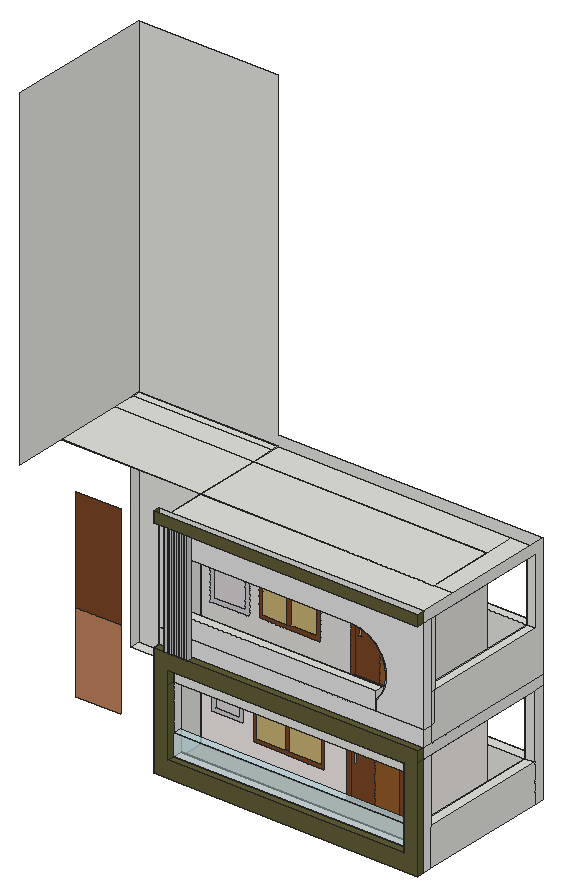
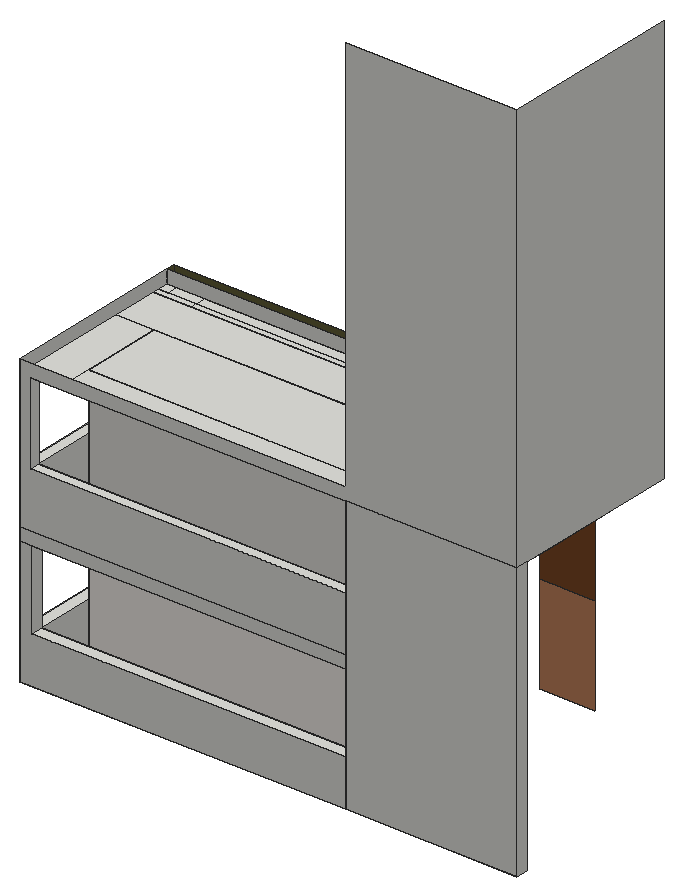
# SketchUp Ruby script. Lengths in inches.
U = 1.inch
M = Sketchup.active_model
def pt(a) = Geom::Point3d.new(a.map { |v| v * U })
def face(e, loops, mat)
  f = e.add_face(loops[0].map { |a| pt(a) })
  loops[1..].each { |l| e.add_face(l.map { |a| pt(a) }).erase! }
  f.material = f.back_material = mat if mat
  f
end
# faces: each face lists its corners as indices into pts; further lists are holes
def faces(e, pts, list, mat = nil) = list.each { |f| face(e, (f[0].is_a?(Array) ? f : [f]).map { |l| l.map { |i| pts[i] } }, mat) }
# xy, xz, yz: faces in a plane at the given z, y or x. An outline is a flat list of corners, or four numbers for a rectangle; further outlines are holes
def ring(l) = l.size == 4 ? [[l[0], l[1]], [l[2], l[1]], [l[2], l[3]], [l[0], l[3]]] : l.each_slice(2).to_a
def flat(e, list, mat, &to3) = list.each { |f| face(e, (f[0].is_a?(Array) ? f : [f]).map { |l| ring(l).map { |u, v| to3.(u, v) } }, mat) }
def xy(e, z, list, mat = nil) = flat(e, list, mat) { |x, y| [x, y, z] }
def xz(e, y, list, mat = nil) = flat(e, list, mat) { |x, z| [x, y, z] }
def yz(e, x, list, mat = nil) = flat(e, list, mat) { |y, z| [x, y, z] }
def lines(e, pts, list) = list.each { |a, b| e.add_line(pt(pts[a]), pt(pts[b])) }
# prism: a flat outline (further loops are holes) pulled along v
def prism(e, loops, v, mat = nil)
  f = face(e, loops, mat); d = Geom::Vector3d.new(v.map { |x| x * U })
  f.pushpull(f.normal.samedirection?(d) ? d.length : -d.length)
end
def box(e, o, s, mat = nil) = prism(e, [[o, [o[0] + s[0], o[1], o[2]], [o[0] + s[0], o[1] + s[1], o[2]], [o[0], o[1] + s[1], o[2]]]], [0, 0, s[2]], mat)
def at(x, y, z, deg = 0) = Geom::Transformation.translation(pt([x, y, z])) * Geom::Transformation.rotation(ORIGIN, Z_AXIS, deg.degrees)
def axes(o, x, y, z) = Geom::Transformation.new([*x, 0, *y, 0, *z, 0, *pt(o).to_a, 1])
def part(name) = M.definitions.add(name)
# library, detail: a bought-in or finely detailed component or shape, given as its bounding box
def library(name, o, s) = part(name).tap { |d| box(d.entities, o, s) }
def detail(e, o, s) = box(e.add_group.entities, o, s)
def put(e, d, t, mat = nil) = e.add_instance(d, t).tap { |i| i.material = mat if mat }
def group(e, t, mat = nil) = e.add_group.tap { |g| g.transformation = t; g.material = mat if mat }.entities
root = M.entities
M.materials.add("[0057_DarkKhaki]").color = [96, 93, 54]
M.materials.add("[Blinds Cellular White]").color = [217, 211, 213]
M.materials.add("[Carpet Diamond Yellow]").color = [226, 217, 124]
M.materials.add("[Carpet Pattern Leaf Squares Tan]").color = [181, 154, 125]
M.materials.add("[Polished Concrete New]").color = [200, 200, 203]
M.materials.add("[Polished Concrete Old]").color = [229, 229, 229]
M.materials.add("[Terrazzo Tile Accent]").color = [224, 221, 217]
M.materials.add("[Translucent Glass Safety]").color = [204, 235, 244]
M.materials["[Translucent Glass Safety]"].alpha = 0.5
M.materials.add("[White Square Tile]").color = [240, 234, 230]
M.materials.add("[Window Covering 02]").color = [199, 178, 115]
M.materials.add("[Wood Floor Light]").color = [204, 176, 127]
M.materials.add("[Wood Floor Parquet]").color = [145, 89, 39]
M.materials.add("[Wood Veneer 01]").color = [120, 70, 37]
M.materials.add("[Wood Veneer 02]").color = [190, 128, 91]
xy(root,354.875,[[386.67,294.37,424.8,314.12],[424.8,294.37,1062.63,314.12],[1062.63,294.37,1099.23,314.12],[386.67,314.12,424.8,338.96],[424.8,314.12,1062.63,338.96],
  [1062.63,314.12,1099.23,338.96],[1072.84,338.96,1072.84,688.57,386.67,688.57,386.67,714.96,1099.23,714.96,1099.23,338.96],[386.67,454.33,997.73,653.02],[11.875,688.57,386.67,714.96]])
xy(root,354.875,[[386.67,338.96,1072.84,338.96,1072.84,688.57,386.67,688.57,386.67,653.02,997.73,653.02,997.73,454.33,386.67,454.33]],"[Carpet Pattern Leaf Squares Tan]")
xy(root,398.5625,[[424.8,314.12,1062.63,338.96]])
xy(root,398.5625,[[424.8,294.37,1062.63,314.12]],"[0057_DarkKhaki]")
xy(root,454.8125,[[424.8,314.12,1062.63,338.96]],"[Translucent Glass Safety]")
xy(root,457.5,[[1072.84,338.96,1099.23,688.57],[386.67,688.57,1072.84,714.96]])
xy(root,579.75,[[424.8,314.12,1062.63,338.96]])
xy(root,616.5625,[[424.8,314.12,1062.63,338.96]])
xy(root,616.5625,[[424.8,294.37,1062.63,314.12]],"[0057_DarkKhaki]")
xy(root,629.6875,[[386.67,338.96,386.67,454.33,997.73,454.33,997.73,714.96,1072.84,714.96,1072.84,688.57,1099.23,688.57,1099.23,338.96],[386.67,454.33,997.73,653.02],[386.67,653.02,997.73,714.96]])
xy(root,657,[[415.15,294.37,424.7,307.59],[427.33,294.37,436.89,307.59],[440.83,294.37,450.39,307.59],[454.9,294.37,464.45,307.59],[467.49,294.37,477.04,307.59],
  [386.67,314.12,386.67,338.96,1075.67,337.88,1099.23,337.88,1099.23,314.12],[1075.67,337.88,1075.67,693,386.67,693,386.67,714.96,1099.23,714.96,1099.23,337.88],[386.67,452.96,1015.29,631.96]])
xy(root,657,[[386.67,294.37,415.15,294.37,415.15,307.59,424.7,307.59,424.7,294.37,427.33,294.37,427.33,307.59,436.89,307.59,436.89,294.37,440.83,294.37,440.83,307.59,450.39,307.59,450.39,294.37,454.9,294.37,454.9,307.59,464.45,307.59,464.45,294.37,467.49,294.37,467.49,307.59,477.04,307.59,477.04,294.37,1099.23,294.37,1099.23,314.12,386.67,314.12]],"[0057_DarkKhaki]")
xy(root,657,[[1075.67,337.88,1075.67,693,386.67,693,386.67,631.96,1015.29,631.96,1015.29,452.96,386.67,452.96,386.67,338.96]],"[Carpet Diamond Yellow]")
xy(root,699.68,[[386.67,314.12,427.13,337.88],[427.13,314.12,903.88,337.98],[903.88,314.12,970.81,337.88],[970.81,314.12,1099.23,337.88],[386.67,337.88,386.67,338.96,427.13,338.89,427.13,337.88],
  [1075.67,337.88,903.88,338.15,903.88,351.68,1099.23,351.68,1099.23,337.88],[903.88,337.88,903.88,338.15,1075.67,337.88],[427.13,338.89,386.67,338.96,386.67,351.68,427.13,351.68]])
xy(root,748.74,[[410.19,314.12,970.81,314.12,970.81,337.88,903.88,337.88,903.88,337.98,427.13,337.98,427.13,337.88,410.19,337.88]])
xy(root,779.4375,[[1075.67,337.88,1099.23,693],[386.67,693,1075.67,714.96]])
xy(root,889.43,[[410.19,314.12,903.88,337.88],[427.13,337.88,903.88,337.98],[427.13,337.98,903.88,351.68]])
xy(root,958.5625,[[386.67,294.37,386.67,314.12,1015.29,314.12,1015.29,294.37,477.04,294.37,477.04,307.59,467.49,307.59,467.49,294.37,464.45,294.37,464.45,307.59,454.9,307.59,454.9,294.37,450.39,294.37,450.39,307.59,440.83,307.59,440.83,294.37,436.89,294.37,436.89,307.59,427.33,307.59,427.33,294.37,424.7,294.37,424.7,307.59,415.15,307.59,415.15,294.37],[415.15,294.37,424.7,307.59],[427.33,294.37,436.89,307.59],[440.83,294.37,450.39,307.59],[454.9,294.37,464.45,307.59],
  [467.49,294.37,477.04,307.59],[1015.29,294.37,1075.67,314.12],[1075.67,294.37,1099.23,314.12],[386.67,314.12,1015.29,314.12,1015.29,337.98,386.67,338.96],[1015.29,314.12,1015.29,337.98,1075.67,337.88,1075.67,314.12],
  [1075.67,314.12,1099.23,337.88],[1075.67,337.88,1099.23,337.88,1099.23,351.68,1015.29,351.68,1015.29,337.98],[1015.29,337.98,386.67,338.96,386.67,351.68,1015.29,351.68],[386.67,351.68,1099.23,452.96],[11.875,452.96,386.67,454.33],
  [386.67,452.96,1015.29,631.96],[1015.29,452.96,1015.29,714.96,1075.67,714.96,1075.67,693,1099.23,693,1099.23,452.96],[11.875,454.33,386.67,631.96],[11.875,631.96,386.67,693],[386.67,631.96,1015.29,714.96],
  [11.875,693,386.67,714.96]])
xz(root,294.37,[[[386.67,354.875,1099.23,657],[424.8,398.5625,1062.63,616.5625]],[386.67,958.5625,1099.23,986.8125]],"[0057_DarkKhaki]")
xz(root,294.37,[[415.15,657,424.7,958.5625],[427.33,657,436.89,958.5625],[440.83,657,450.39,958.5625],[454.9,657,464.45,958.5625],[467.49,657,477.04,958.5625]],"[Polished Concrete New]")
xz(root,307.59,[[415.15,657,424.7,958.5625],[427.33,657,436.89,958.5625],[440.83,657,450.39,958.5625],[454.9,657,464.45,958.5625],[467.49,657,477.04,958.5625]])
xz(root,314.12,[[424.8,579.75,1062.63,616.5625],[386.67,958.5625,1099.23,986.8125]])
xz(root,314.12,[[386.67,657,1099.23,699.68],[386.67,699.68,970.81,699.68,970.81,748.74,410.19,748.74,410.19,889.43,903.88,889.43,928.43,886.2,951.31,876.72,970.96,861.64,986.04,841.99,995.52,819.11,998.75,794.55,995.52,770,986.04,747.12,970.96,727.47,970.81,727.35,970.81,699.68,1099.23,699.68,1099.23,958.5625,386.67,958.5625]],"[Polished Concrete Old]")
xz(root,314.12,[[424.8,398.5625,1062.63,454.8125]],"[Translucent Glass Safety]")
xz(root,314.12,[[163.125,665.78,282.875,947.1]],"[Wood Veneer 01]")
xz(root,314.12,[[163.125,450.91,282.875,665.78]],"[Wood Veneer 02]")
xz(root,337.88,[[1075.67,657,1099.23,699.68],[903.88,699.68,903.88,748.74,970.81,748.74,970.81,727.35,951.31,712.39,928.44,702.91,928.43,702.91],[903.88,699.68,928.43,702.91,970.81,702.91,970.81,699.68],[1075.67,699.68,1099.23,779.4375],[928.44,702.91,951.31,712.39,970.81,727.35,970.81,702.91],
  [410.19,748.74,427.13,889.43],[1075.67,779.4375,1099.23,958.5625]])
xz(root,337.98,[[427.13,699.68,903.88,748.74]])
xz(root,338.96,[[386.67,354.875,424.8,629.6875],[424.8,354.875,1062.63,398.5625],[1062.63,354.875,1072.84,629.6875],[1072.84,354.875,1099.23,457.5],[1072.84,457.5,1099.23,629.6875],
  [424.8,579.75,1062.63,616.5625],[424.8,616.5625,1062.63,629.6875]])
xz(root,338.96,[[424.8,398.5625,1062.63,454.8125]],"[Translucent Glass Safety]")
xz(root,351.68,[[386.67,699.68,386.67,958.5625,1099.23,958.5625,1099.23,699.68,903.88,699.68,928.43,702.91,951.31,712.39,970.96,727.47,986.04,747.12,995.52,770,998.75,794.55,995.52,819.11,986.04,841.99,970.96,861.64,951.31,876.72,928.43,886.2,903.88,889.43,427.13,889.43,427.13,699.68]])
xz(root,452.96,[[426.7,722.16,505.57,891.53]],"[Blinds Cellular White]")
xz(root,452.96,[[[412.01,707.47,520.26,906.22],[426.7,722.16,505.57,891.53]]],"[Polished Concrete New]")
xz(root,452.96,[[[386.67,657,791.59,657,791.59,909.62,947.71,909.62,947.71,657,1015.29,657,1015.29,958.5625,386.67,958.5625],[543.9,713.72,712.34,916.97],[412.01,707.47,520.26,906.22]]],"[Terrazzo Tile Accent]")
xz(root,452.96,[[555.49,725.3125,620.61,905.39],[631.375,725.3125,700.75,905.39]],"[Window Covering 02]")
xz(root,452.96,[[813.71,765.94,820.84,802]],"[Wood Floor Light]")
xz(root,452.96,[[869.65,669.16,935.55,897.45]],"[Wood Floor Parquet]")
xz(root,452.96,[[[791.59,657,947.71,909.62],[803.75,669.16,935.55,897.45]],[[803.75,669.16,869.65,897.45],[813.71,765.94,820.84,802]],[[543.9,713.72,712.34,916.97],[555.49,725.3125,700.75,905.39]],[620.61,725.3125,631.375,905.39]],"[Wood Veneer 01]")
xz(root,454.33,[[427.2,455.19,491.51,583.375]],"[Blinds Cellular White]")
xz(root,454.33,[[[417.48,445.47,501.23,593.1],[427.2,455.19,491.51,583.375]]],"[Polished Concrete New]")
xz(root,454.33,[[[386.67,354.875,780.78,354.875,780.78,598.89,931.59,598.89,931.59,354.875,997.73,354.875,997.73,629.6875,386.67,629.6875],[527.13,407.43,722.26,594.5],[417.48,445.47,501.23,593.1]]],"[White Square Tile]")
xz(root,454.33,[[538.625,418.92,614.39,583],[627.28,418.92,710.77,583]],"[Window Covering 02]")
xz(root,454.33,[[798.35,452.18,806.16,494.55]],"[Wood Floor Light]")
xz(root,454.33,[[856.18,364.13,922.33,589.64]],"[Wood Floor Parquet]")
xz(root,454.33,[[[780.78,354.875,931.59,598.89],[790.03,364.13,922.33,589.64]],[[790.03,364.13,856.18,589.64],[798.35,452.18,806.16,494.55]],[[527.13,407.43,722.26,594.5],[538.625,418.92,710.77,583]],[614.39,418.92,627.28,583]],"[Wood Veneer 01]")
xz(root,631.96,[[386.67,657,1015.29,958.5625]],"[Terrazzo Tile Accent]")
xz(root,653.02,[[386.67,354.875,997.73,629.6875]],"[White Square Tile]")
xz(root,688.57,[[386.67,354.875,1072.84,457.5],[1072.84,457.5,1099.23,629.6875]])
xz(root,693,[[386.67,657,1075.67,779.4375],[1075.67,779.4375,1099.23,958.5625]])
xz(root,714.96,[[11.875,354.875,386.67,958.5625],[386.67,354.875,386.67,457.5,1072.84,457.5,1072.84,629.6875,1099.23,629.6875,1099.23,354.875],[386.67,629.6875,1099.23,657],[386.67,657,386.67,779.4375,1075.67,779.4375,1075.67,958.5625,11.875,958.5625,11.875,1855.8125,386.67,1855.8125,386.67,986.8125,1099.23,986.8125,1099.23,657]])
yz(root,11.875,[[688.57,354.875,714.96,958.5625],[314.12,958.5625,714.96,1855.8125]])
yz(root,386.67,[[314.12,354.875,338.96,657],[338.96,354.875,454.33,629.6875],[454.33,354.875,653.02,629.6875],[653.02,354.875,688.57,354.875,688.57,457.5,714.96,457.5,714.96,629.6875,653.02,629.6875],[688.57,354.875,714.96,457.5],
  [338.96,629.6875,454.33,657],[454.33,629.6875,653.02,657],[653.02,629.6875,714.96,657],[314.12,657,338.96,699.68],[338.96,657,452.96,657,452.96,958.5625,351.68,958.5625,351.68,699.68,338.96,699.68],
  [452.96,657,454.33,958.5625],[454.33,657,631.96,958.5625],[631.96,657,693,958.5625],[693,657,714.96,779.4375],[314.12,699.68,337.88,958.5625],
  [337.88,699.68,338.96,958.5625],[338.96,699.68,351.68,958.5625],[693,779.4375,714.96,958.5625]])
yz(root,386.67,[[294.37,354.875,314.12,657],[294.37,958.5625,314.12,986.8125]],"[0057_DarkKhaki]")
yz(root,410.19,[[314.12,748.74,337.88,889.43]])
yz(root,415.15,[[294.37,657,307.59,958.5625]],"[Polished Concrete New]")
yz(root,424.7,[[294.37,657,307.59,958.5625]],"[Polished Concrete New]")
yz(root,424.8,[[314.12,398.5625,338.96,454.8125],[314.12,579.75,338.96,616.5625]])
yz(root,424.8,[[294.37,398.5625,314.12,579.75],[294.37,579.75,314.12,616.5625]],"[0057_DarkKhaki]")
yz(root,424.8,[[314.12,454.8125,338.96,579.75]],"[Polished Concrete Old]")
yz(root,427.13,[[337.88,699.68,337.98,748.74],[337.98,699.68,351.68,889.43],[337.88,748.74,337.98,889.43]])
yz(root,427.33,[[294.37,657,307.59,958.5625]],"[Polished Concrete New]")
yz(root,436.89,[[294.37,657,307.59,958.5625]],"[Polished Concrete New]")
yz(root,440.83,[[294.37,657,307.59,958.5625]],"[Polished Concrete New]")
yz(root,450.39,[[294.37,657,307.59,958.5625]],"[Polished Concrete New]")
yz(root,454.9,[[294.37,657,307.59,958.5625]],"[Polished Concrete New]")
yz(root,464.45,[[294.37,657,307.59,958.5625]],"[Polished Concrete New]")
yz(root,467.49,[[294.37,657,307.59,958.5625]],"[Polished Concrete New]")
yz(root,477.04,[[294.37,657,307.59,958.5625]],"[Polished Concrete New]")
yz(root,903.88,[[337.88,699.68,337.98,748.74]])
yz(root,970.81,[[314.12,699.68,337.88,748.74]])
yz(root,997.73,[[454.33,354.875,653.02,629.6875]],"[White Square Tile]")
yz(root,1015.29,[[452.96,657,631.96,958.5625]],"[Terrazzo Tile Accent]")
yz(root,1062.63,[[314.12,398.5625,338.96,454.8125],[314.12,579.75,338.96,616.5625]])
yz(root,1062.63,[[294.37,398.5625,314.12,579.75],[294.37,579.75,314.12,616.5625]],"[0057_DarkKhaki]")
yz(root,1062.63,[[314.12,454.8125,338.96,579.75]],"[Polished Concrete Old]")
yz(root,1072.84,[[338.96,354.875,688.57,457.5],[688.57,457.5,714.96,629.6875]])
yz(root,1075.67,[[337.88,657,693,779.4375],[693,779.4375,714.96,958.5625]])
yz(root,1099.23,[[338.96,354.875,688.57,457.5],[688.57,354.875,714.96,629.6875],[314.12,629.6875,714.96,657],[314.12,657,337.88,699.68],[337.88,657,714.96,657,714.96,986.8125,314.12,986.8125,314.12,958.5625,693,958.5625,693,779.4375,351.68,779.4375,351.68,699.68,337.88,699.68],
  [337.88,699.68,351.68,779.4375],[337.88,779.4375,351.68,958.5625]])
yz(root,1099.23,[[294.37,354.875,314.12,629.6875],[294.37,629.6875,314.12,657],[294.37,958.5625,314.12,986.8125]],"[0057_DarkKhaki]")
yz(root,1099.23,[[314.12,354.875,338.96,629.6875],[314.12,699.68,337.88,958.5625]],"[Polished Concrete Old]")
p = [[1075.67,337.88,657],[386.67,338.96,657],[386.67,338.96,699.68],[427.13,338.89,699.68],[903.88,338.15,699.68],[1075.67,337.88,699.68],
  [903.88,337.98,699.68],[903.88,337.88,699.68],[928.43,337.88,702.91],[928.43,337.98,702.91],[928.43,351.68,702.91],[903.88,351.68,699.68],
  [928.44,337.88,702.91],[951.31,337.88,712.39],[951.31,337.98,712.39],[951.31,351.68,712.39],[970.81,337.88,727.35],[970.96,337.88,727.47],
  [970.96,337.98,727.47],[970.96,351.68,727.47],[970.96,314.12,727.47],[986.04,314.12,747.12],[986.04,337.88,747.12],[986.04,337.98,747.12],
  [986.04,351.68,747.12],[995.52,314.12,770],[995.52,337.88,770],[995.52,337.98,770],[995.52,351.68,770],[998.75,314.12,794.55],
  [998.75,337.88,794.55],[998.75,337.98,794.55],[998.75,351.68,794.55],[995.52,314.12,819.11],[995.52,337.88,819.11],[995.52,337.98,819.11],
  [995.52,351.68,819.11],[986.04,314.12,841.99],[986.04,337.88,841.99],[986.04,337.98,841.99],[986.04,351.68,841.99],[970.96,314.12,861.64],
  [970.96,337.88,861.64],[970.96,337.98,861.64],[970.96,351.68,861.64],[951.31,314.12,876.72],[951.31,337.88,876.72],[951.31,337.98,876.72],
  [951.31,351.68,876.72],[928.43,314.12,886.2],[928.43,337.88,886.2],[928.43,337.98,886.2],[928.43,351.68,886.2],[903.88,314.12,889.43],
  [903.88,337.88,889.43],[903.88,337.98,889.43],[903.88,351.68,889.43]]
faces(root,p,[[0,1,2,3,4,5],[6,7,8,9],[4,6,9,10,11],[9,8,12,13,14],[10,9,14,15],[14,13,16,17,18],[15,14,18,19],[20,21,22,17],
  [18,17,22,23],[19,18,23,24],[21,25,26,22],[23,22,26,27],[24,23,27,28],[25,29,30,26],[27,26,30,31],[28,27,31,32],
  [29,33,34,30],[31,30,34,35],[32,31,35,36],[33,37,38,34],[35,34,38,39],[36,35,39,40],[37,41,42,38],[39,38,42,43],
  [40,39,43,44],[41,45,46,42],[43,42,46,47],[44,43,47,48],[45,49,50,46],[47,46,50,51],[48,47,51,52],[49,53,54,50],
  [51,50,54,55],[52,51,55,56]])
